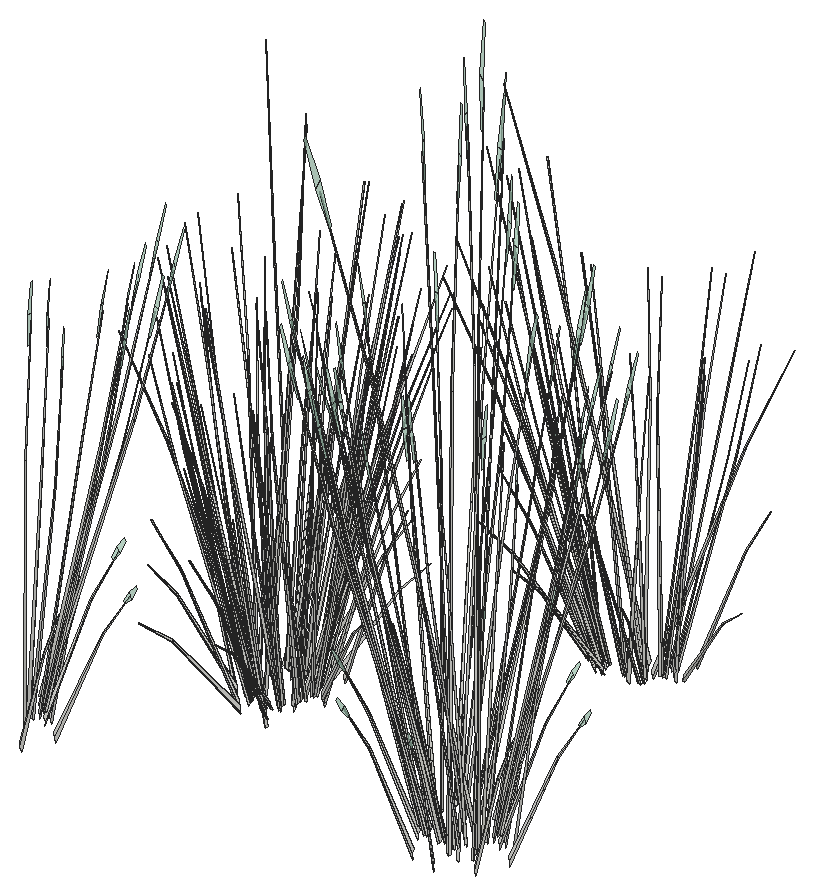
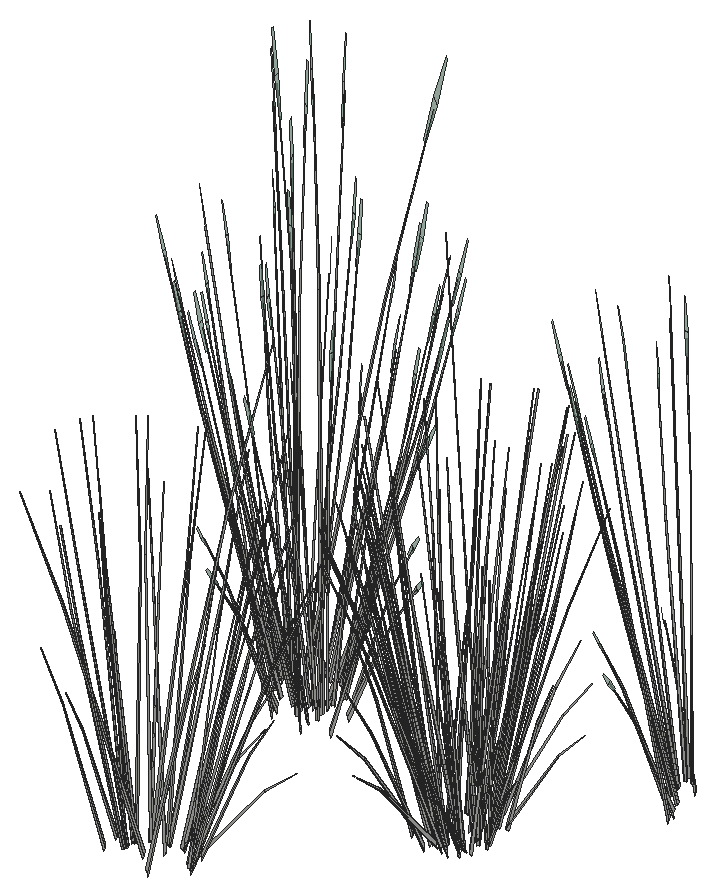
# SketchUp Ruby script. Lengths in inches.
U = 1.inch
M = Sketchup.active_model
def pt(a) = Geom::Point3d.new(a.map { |v| v * U })
def face(e, loops, mat)
  f = e.add_face(loops[0].map { |a| pt(a) })
  loops[1..].each { |l| e.add_face(l.map { |a| pt(a) }).erase! }
  f.material = f.back_material = mat if mat
  f
end
# faces: each face lists its corners as indices into pts; further lists are holes
def faces(e, pts, list, mat = nil) = list.each { |f| face(e, (f[0].is_a?(Array) ? f : [f]).map { |l| l.map { |i| pts[i] } }, mat) }
# xy, xz, yz: faces in a plane at the given z, y or x. An outline is a flat list of corners, or four numbers for a rectangle; further outlines are holes
def ring(l) = l.size == 4 ? [[l[0], l[1]], [l[2], l[1]], [l[2], l[3]], [l[0], l[3]]] : l.each_slice(2).to_a
def flat(e, list, mat, &to3) = list.each { |f| face(e, (f[0].is_a?(Array) ? f : [f]).map { |l| ring(l).map { |u, v| to3.(u, v) } }, mat) }
def xy(e, z, list, mat = nil) = flat(e, list, mat) { |x, y| [x, y, z] }
def xz(e, y, list, mat = nil) = flat(e, list, mat) { |x, z| [x, y, z] }
def yz(e, x, list, mat = nil) = flat(e, list, mat) { |y, z| [x, y, z] }
def lines(e, pts, list) = list.each { |a, b| e.add_line(pt(pts[a]), pt(pts[b])) }
# prism: a flat outline (further loops are holes) pulled along v
def prism(e, loops, v, mat = nil)
  f = face(e, loops, mat); d = Geom::Vector3d.new(v.map { |x| x * U })
  f.pushpull(f.normal.samedirection?(d) ? d.length : -d.length)
end
def box(e, o, s, mat = nil) = prism(e, [[o, [o[0] + s[0], o[1], o[2]], [o[0] + s[0], o[1] + s[1], o[2]], [o[0], o[1] + s[1], o[2]]]], [0, 0, s[2]], mat)
def at(x, y, z, deg = 0) = Geom::Transformation.translation(pt([x, y, z])) * Geom::Transformation.rotation(ORIGIN, Z_AXIS, deg.degrees)
def axes(o, x, y, z) = Geom::Transformation.new([*x, 0, *y, 0, *z, 0, *pt(o).to_a, 1])
def part(name) = M.definitions.add(name)
# library, detail: a bought-in or finely detailed component or shape, given as its bounding box
def library(name, o, s) = part(name).tap { |d| box(d.entities, o, s) }
def detail(e, o, s) = box(e.add_group.entities, o, s)
def put(e, d, t, mat = nil) = e.add_instance(d, t).tap { |i| i.material = mat if mat }
def group(e, t, mat = nil) = e.add_group.tap { |g| g.transformation = t; g.material = mat if mat }.entities
root = M.entities
M.materials.add("LightPink_Translucent").color = [175, 214, 192]
M.materials["LightPink_Translucent"].alpha = 0.75
c1 = part("blade")
p = [[2.15,0.21,22],[0,0.17,0],[0.09,0.45,0],[2.18,0.31,22],[2.29,0.31,22],[0.38,0.45,0],
  [2.48,0.24,33],[2.49,0.24,33],[2.48,0.22,33]]
faces(c1.entities,p,[[0,1,2,3],[4,5,2,3],[6,3,4,7],[8,0,3,6]])
c2 = part("seeds")
p = [[0.3,-0.1,1.38],[-0.01,-0.03,1.59],[-0.01,-0.03,0.03],[0.14,-0.07,-0.07],[0.29,-0.03,3],[0.15,0.01,3.11]]
faces(c2.entities,p,[[0,1,2,3],[1,0,4,5]],"LightPink_Translucent")
c3 = part("blade with seeds")
put(c3.entities,c1,at(0,0,0))
put(c3.entities,c2,axes([2.4,0.25,30.99],[1.5799,-0.05474,1.17369],[-0.12525,1.92788,0.29478],[-0.07173,-0.02425,1.56792]))
c4 = part("blade with seeds\#1")
put(c4.entities,c1,at(0,0,0))
put(root,c3,axes([465.16,230.9,141.8],[0.24965,-0.35138,-0.64651],[0.43748,0.24972,0.07802],[0.14906,-0.12731,0.91455]))
put(root,c3,axes([465.14,230.74,141.52],[-0.12278,-0.40663,-0.465],[0.46497,-0.07113,-0.36018],[0.13325,-0.10922,0.88973]))
put(root,c3,axes([465.71,229.93,139.78],[-0.15919,0.2267,1.04523],[-0.13683,-0.30457,0.76796],[0.13148,-0.07632,0.23022]))
put(root,c3,axes([465.49,230.78,141.38],[0.41603,-0.06364,-0.32227],[0.10985,0.36383,0.41605],[0.11922,-0.09772,0.79608]))
put(root,c3,axes([465.36,231.64,141.52],[0.12948,-0.40508,-0.465],[0.44393,0.13885,-0.36018],[0.17873,-0.03714,0.88973]))
put(root,c3,axes([465.28,231.79,141.8],[0.41997,-0.19668,-0.64651],[0.23405,0.40486,0.07802],[0.20292,-0.04599,0.91455]))
put(root,c3,axes([491.3125,234.65,141.7],[-0.22811,-0.3621,-0.64651],[0.46957,-0.2018,0.07802],[-0.05334,-0.17496,0.91455]))
put(root,c3,axes([492.26,235,141.7],[0.01244,-0.41193,-0.64651],[0.52368,0.02767,0.07802],[0.05527,-0.17451,0.91455]))
put(root,c3,axes([491.36,234.34,141.29],[0.14409,-0.34247,-0.32227],[0.42037,0.09989,0.41605],[-0.03855,-0.13788,0.79608]))
put(root,c3,axes([465.63,231.82,141.38],[0.3972,0.12423,-0.32227],[-0.11585,0.36244,0.41605],[0.15992,-0.03323,0.79608]))
put(root,c3,axes([491.14,234.57,141.43],[-0.46982,-0.11164,-0.465],[0.16104,-0.38276,-0.36018],[-0.04308,-0.1541,0.88973]))
put(root,c3,axes([491.43,233.62,139.6875],[0.06131,0.25968,1.04523],[-0.34012,-0.14383,0.76796],[0.0366,-0.13297,0.23022]))
put(root,c3,axes([492.16,234.86,141.43],[-0.34214,-0.29922,-0.465],[0.36143,-0.26205,-0.36018],[0.05206,-0.15203,0.88973]))
put(root,c3,axes([492.48,234.75,141.29],[0.32338,-0.23447,-0.32227],[0.30612,0.26773,0.41605],[0.04658,-0.13603,0.79608]))
put(root,c3,axes([489.68,233.93,139.6875],[0.24931,0.155,1.04523],[-0.36309,0.09317,0.76796],[-0.07769,-0.11912,0.23022]))
put(root,c3,axes([490.29,234.75,141.7],[-0.40754,-0.21525,-0.64651],[0.28963,-0.37719,0.07802],[-0.14765,-0.12852,0.91455]))
put(root,c3,axes([490.14,234.47,141.29],[-0.07382,-0.3587,-0.32227],[0.42197,-0.09472,0.41605],[-0.11334,-0.10279,0.79608]))
put(root,c3,axes([466.47,231.9,139.78],[-0.2953,0.07352,1.04523],[0.139,-0.30384,0.76796],[0.15666,0.02079,0.23022]))
put(root,c3,axes([490.1,234.76,141.43],[-0.47162,0.10586,-0.465],[-0.0825,-0.4009,-0.36018],[-0.12667,-0.11489,0.88973]))
put(root,c3,axes([492.88,235.72,141.7],[0.24965,-0.35138,-0.64651],[0.43748,0.24972,0.07802],[0.14906,-0.12731,0.91455]))
put(root,c3,axes([492.87,235.55,141.43],[-0.12278,-0.40663,-0.465],[0.46497,-0.07113,-0.36018],[0.13325,-0.10922,0.88973]))
put(root,c3,axes([491.26,237.19,140.2],[0.41302,0.17958,1.37647],[-0.40462,0.38687,0.54432],[-0.18124,-0.22929,1.15394]))
put(root,c3,axes([464.86,232.6,141.8],[0.47777,0.01072,-0.64651],[-0.03209,0.45152,0.07802],[0.2024,0.04765,0.91455]))
put(root,c3,axes([493.4375,234.74,139.6875],[-0.15919,0.2267,1.04523],[-0.13683,-0.30457,0.76796],[0.13148,-0.07632,0.23022]))
put(root,c3,axes([493.21,235.6,141.29],[0.41603,-0.06364,-0.32227],[0.10985,0.36383,0.41605],[0.11922,-0.09772,0.79608]))
put(root,c3,axes([489.17,235.1,141.29],[-0.27194,-0.27882,-0.32227],[0.31051,-0.26394,0.41605],[-0.15777,-0.04016,0.79608]))
put(root,c3,axes([465.15,232.79,141.38],[0.27194,0.27882,-0.32227],[-0.31051,0.26394,0.41605],[0.15777,0.04016,0.79608]))
put(root,c3,axes([489.45,235.28,141.7],[-0.47777,-0.01072,-0.64651],[0.03209,-0.45152,0.07802],[-0.2024,-0.04765,0.91455]))
put(root,c3,axes([464.83,232.95,139.78],[-0.2691,-0.12805,1.04523],[0.34747,-0.13011,0.76796],[0.09372,0.11021,0.23022]))
put(root,c3,axes([489.3,235.375,141.43],[-0.34704,0.29499,-0.465],[-0.30393,-0.31162,-0.36018],[-0.17633,-0.04488,0.88973]))
put(root,c3,axes([488.51,235.76,139.6875],[0.30513,-0.03187,1.04523],[-0.19355,0.28077,0.76796],[-0.15079,-0.04212,0.23022]))
put(root,c3,axes([490.67,236.02,139.64],[-0.519,0.02749,0.40713],[-0.04694,-0.45634,-0.19594],[0.09291,-0.04625,1.30716]))
put(root,c3,axes([464.22,233.125,141.52],[0.47162,-0.10586,-0.465],[0.0825,0.4009,-0.36018],[0.12667,0.11489,0.88973]))
put(root,c3,axes([493.08,236.46,141.43],[0.12948,-0.40508,-0.465],[0.44393,0.13885,-0.36018],[0.17873,-0.03714,0.88973]))
put(root,c3,axes([464.875,233.53,139.69],[-0.30649,-0.01397,0.95605],[0.2024,-0.29664,0.52785],[0.12108,0.10539,0.74993]))
put(root,c3,axes([490.55,236.58,139.64],[-0.23189,0.40128,0.40713],[-0.48183,-0.19312,-0.19594],[0,-0.0925,1.30716]))
put(root,c3,axes([493,236.6,141.7],[0.41997,-0.19668,-0.64651],[0.23405,0.40486,0.07802],[0.20292,-0.04599,0.91455]))
put(root,c3,axes([491.29,235.84,139.64],[-0.28711,-0.37379,0.40713],[0.43489,-0.26322,-0.19594],[0.09291,0.04625,1.30716]))
put(root,c3,axes([493.36,236.64,141.29],[0.3972,0.12423,-0.32227],[-0.11585,0.36244,0.41605],[0.15992,-0.03323,0.79608]))
put(root,c3,axes([488.6875,236.0625,141.29],[-0.3972,-0.12423,-0.32227],[0.11585,-0.36244,0.41605],[-0.15992,0.03323,0.79608]))
put(root,c4,axes([473.13,239.73,140.59],[-0.05804,-0.06898,1.43516],[-0.35603,0.0883,-0.22697],[-0.0675,-0.17309,0.1151]))
put(root,c3,axes([489.9,236,140.21],[0.13585,-0.06442,1.61128],[0.04685,0.4498,0.1261],[-0.29426,0.05969,0.57588]))
put(root,c3,axes([494.2,236.71,139.6875],[-0.2953,0.07352,1.04523],[0.139,-0.30384,0.76796],[0.15666,0.02079,0.23022]))
put(root,c4,axes([474.7,240.09,140.58],[-0.03336,0.04495,1.45516],[-0.35758,-0.09833,-0.1375],[-0.02285,-0.17707,0.25751]))
put(root,c4,axes([473.15,241.95,139.9],[0.00863,0.2062,1.40588],[-0.37404,-0.13679,0.11368],[0.02314,-0.29386,0.601]))
put(root,c3,axes([491.79,236.21,139.64],[0.23189,-0.40128,0.40713],[0.48183,0.19312,-0.19594],[0,0.0925,1.30716]))
put(root,c3,axes([488.96,236.25,141.43],[-0.12948,0.40508,-0.465],[-0.44393,-0.13885,-0.36018],[-0.17873,0.03714,0.88973]))
put(root,c3,axes([493.6875,237.65,140.75],[-0.09148,-0.37435,-0.03177],[0.43236,-0.08606,-0.14407],[0.09029,0.02373,0.47519]))
put(root,c4,axes([473.53,240.82,140.43],[0.1063,-0.41315,-0.29052],[0.31012,0.1205,0.37506],[-0.02844,-0.16634,0.71765]))
put(root,c3,axes([491.67,236.76,139.64],[0.519,-0.02749,0.40713],[0.04694,0.45634,-0.19594],[-0.09291,0.04625,1.30716]))
put(root,c4,axes([474.16,241.21,140.59],[-0.00644,-0.10664,1.43516],[-0.29603,-0.29251,-0.22697],[0.03908,-0.18969,0.1151]))
put(root,c4,axes([473.67,241.08,140.85],[-0.34504,0.25013,-0.09976],[-0.16956,-0.44394,-0.55369],[-0.04552,-0.18708,0.84132]))
put(root,c4,axes([473.57,240.92,140.6],[0.34743,0.14045,0.39379],[-0.1188,0.46175,0.3247],[-0.02088,-0.18159,0.81485]))
put(root,c4,axes([474.39,241.65,140.85],[-0.38751,-0.02662,-0.09976],[0.01059,-0.50399,-0.55369],[0.02692,-0.19411,0.84132]))
put(root,c4,axes([473.66,240.88,140.6],[0.25981,-0.18259,0.05275],[0.12717,0.33295,0.41527],[-0.02509,-0.14677,0.63322]))
put(root,c4,axes([472.76,239.97,140.58],[-0.00289,0.06493,1.45516],[-0.31009,0.26964,-0.1375],[-0.10196,-0.10828,0.25751]))
put(root,c4,axes([472.64,240.97,140.43],[-0.05446,-0.43273,-0.29052],[0.31131,-0.11427,0.37506],[-0.08362,-0.12401,0.71765]))
put(root,c4,axes([474.36,241.32,140.43],[0.23857,-0.28286,-0.29052],[0.22584,0.32298,0.37506],[0.03436,-0.1641,0.71765]))
put(root,c3,axes([492.59,237.42,141.7],[0.47777,0.01072,-0.64651],[-0.03209,0.45152,0.07802],[0.2024,0.04765,0.91455]))
put(root,c4,axes([473.75,242.34,139.9],[-0.06565,0.18466,1.40588],[-0.27542,-0.38215,0.11368],[0.12424,-0.23818,0.601]))
put(root,c4,axes([472.71,241.03,140.6],[0.35069,-0.12329,0.39379],[0.06086,0.48364,0.3247],[-0.08248,-0.14254,0.81485]))
put(root,c4,axes([472.77,240.93,140.6],[0.16025,-0.34128,0.05275],[0.22821,0.1987,0.41527],[-0.07378,-0.10942,0.63322]))
put(root,c3,axes([488.08,237.98,139.6875],[0.19918,-0.20183,1.04523],[0.0786,0.31952,0.76796],[-0.14394,0.05721,0.23022]))
put(root,c3,axes([492.875,237.61,141.29],[0.27194,0.27882,-0.32227],[-0.31051,0.26394,0.41605],[0.15777,0.04016,0.79608]))
put(root,c3,axes([488.83,237.11,141.29],[-0.41603,0.06364,-0.32227],[-0.10985,-0.36383,0.41605],[-0.11922,0.09772,0.79608]))
put(root,c4,axes([474.4,240.48,139.94],[-0.32031,0.09515,-0.02864],[-0.07364,-0.44972,-0.12987],[0.02031,-0.09391,0.42837]))
put(root,c4,axes([474.36,241.43,140.6],[0.25108,0.36656,0.39379],[-0.26664,0.31614,0.3247],[0.04631,-0.17198,0.81485]))
put(root,c4,axes([474.45,241.47,140.6],[0.28975,0.02503,0.05275],[-0.00794,0.378,0.41527],[0.03032,-0.1448,0.63322]))
put(root,c4,axes([472.85,241.1,140.85],[-0.21011,0.45986,-0.09976],[-0.30427,-0.26493,-0.55369],[-0.10577,-0.12992,0.84132]))
put(root,c3,axes([492.56,237.77,139.6875],[-0.2691,-0.12805,1.04523],[0.34747,-0.13011,0.76796],[0.09372,0.11021,0.23022]))
put(root,c4,axes([474.81,242.64,140.85],[-0.32616,-0.29624,-0.09976],[0.1879,-0.42901,-0.55369],[0.09215,-0.14913,0.84132]))
put(root,c3,axes([489.18,237.15,141.43],[0.12278,0.40663,-0.465],[-0.46497,0.07113,-0.36018],[-0.13325,0.10922,0.88973]))
put(root,c3,axes([491.9,236.33,139.76],[-0.01306,-0.4193,1.28558],[0.59089,0.10869,0.54432],[-0.13975,0.22943,1.21348]))
put(root,c4,axes([471.95,242.57,139.9],[0.13097,0.09256,1.40588],[-0.27104,0.38832,0.11368],[-0.16893,-0.17518,0.601]))
put(root,c3,axes([491.95,237.94,141.43],[0.47162,-0.10586,-0.465],[0.0825,0.4009,-0.36018],[0.12667,0.11489,0.88973]))
put(root,c3,axes([492.6,238.35,139.6],[-0.30649,-0.01397,0.95605],[0.2024,-0.29664,0.52785],[0.12108,0.10539,0.74993]))
put(root,c4,axes([471.58,241.2,140.59],[-0.07584,0.0048,1.43516],[-0.21918,0.40531,-0.22697],[-0.13286,-0.06266,0.1151]))
put(root,c4,axes([472,241.74,140.6],[0.25999,-0.354,0.39379],[0.22422,0.37594,0.3247],[-0.12198,-0.0653,0.81485]))
put(root,c4,axes([472.02,241.61,140.6],[0.01775,-0.40853,0.05275],[0.2681,0.0112,0.41527],[-0.1027,-0.04275,0.63322]))
put(root,c4,axes([472.89,242.3,140.39],[-0.19798,0.42958,1.1344],[-0.30825,-0.45359,0.48946],[0.18577,-0.1386,1.09651]))
put(root,c4,axes([471.92,241.73,140.43],[-0.20062,-0.33637,-0.29052],[0.22908,-0.31842,0.37506],[-0.11639,-0.04845,0.71765]))
put(root,c4,axes([475.08,243.02,140.58],[-0.04613,-0.00147,1.45516],[-0.20353,-0.42603,-0.1375],[0.07265,-0.14798,0.25751]))
put(root,c3,axes([489.56,237.95,141.29],[-0.32338,0.23447,-0.32227],[-0.30612,-0.26773,0.41605],[-0.04658,0.13603,0.79608]))
put(root,c3,axes([489.77,238.86,139.6875],[-0.01237,-0.2648,1.04523],[0.30908,0.18886,0.76796],[-0.06079,0.12621,0.23022]))
put(root,c3,axes([489.89,237.84,141.72],[0.34214,0.29922,-0.51615],[-0.36143,0.26205,-0.3998],[-0.05206,0.15203,0.9876]))
put(root,c4,axes([474.13,243.1,139.9],[-0.12234,0.11364,1.40588],[-0.103,-0.52511,0.11368],[0.19206,-0.11868,0.601]))
put(root,c4,axes([474.86,242.43,140.6],[0.08745,0.49445,0.39379],[-0.34303,0.08581,0.3247],[0.1011,-0.11629,0.81485]))
put(root,c3,axes([490.9,238.13,141.43],[0.46982,0.11164,-0.465],[-0.16104,0.38276,-0.36018],[0.04308,0.1541,0.88973]))
put(root,c4,axes([474.93,242.53,140.6],[0.24206,0.22594,0.05275],[-0.14093,0.32175,0.41527],[0.07761,-0.10402,0.63322]))
put(root,c3,axes([490.6875,238.37,141.29],[-0.14409,0.34247,-0.32227],[-0.42037,-0.09989,0.41605],[0.03855,0.13788,0.79608]))
put(root,c3,axes([489.78,237.7,142.03],[-0.01244,0.41193,-0.71763],[-0.52368,-0.02767,0.0866],[-0.05527,0.17451,1.01516]))
put(root,c4,axes([472.15,241.7,140.85],[-0.01888,0.54637,-0.09976],[-0.35746,-0.01493,-0.55369],[-0.13767,-0.03795,0.84132]))
put(root,c3,axes([490.73,238.06,141.7],[0.22811,0.3621,-0.64651],[-0.46957,0.2018,0.07802],[0.05334,0.17496,0.91455]))
put(root,c4,axes([471.31,241.31,140.58],[0.0291,0.05049,1.45516],[-0.09819,0.49465,-0.1375],[-0.12701,0.01791,0.25751]))
put(root,c4,axes([474.82,243.79,140.85],[-0.17741,-0.48648,-0.09976],[0.31487,-0.23906,-0.55369],[0.13269,-0.06419,0.84132]))
put(root,c3,axes([489.6,238.28,140.23],[0.0105,-0.22989,1.40454],[0.4723,0.12143,0.19409],[-0.04092,0.24501,0.66323]))
put(root,c4,axes([471.63,242.85,140.6],[0.09962,-0.48986,0.39379],[0.3275,0.16751,0.3247],[-0.12879,0.02944,0.81485]))
put(root,c4,axes([471.61,242.72,140.6],[-0.1295,-0.36632,0.05275],[0.23615,-0.1793,0.41527],[-0.1041,0.03538,0.63322]))
put(root,c4,axes([475.53,243.91,140.59],[0.06136,-0.06302,1.43516],[0.02411,-0.50855,-0.22697],[0.13532,-0.05114,0.1151]))
put(root,c4,axes([471.5625,242.9,140.43],[-0.29303,-0.14987,-0.29052],[0.08547,-0.43725,0.37506],[-0.11798,0.04009,0.71765]))
put(root,c4,axes([475.01,243.6,140.43],[0.29303,0.14987,-0.29052],[-0.08547,0.43725,0.37506],[0.11798,-0.04009,0.71765]))
put(root,c4,axes([474.97,243.78,140.6],[0.1295,0.36632,0.05275],[-0.23615,0.1793,0.41527],[0.1041,-0.03538,0.63322]))
put(root,c4,axes([474.19,244.03,139.9],[-0.14625,0.01217,1.40588],[0.09702,-0.52737,0.11368],[0.20842,0.03262,0.601]))
put(root,c4,axes([471.75,242.71,140.85],[0.17741,0.48648,-0.09976],[-0.31487,0.23906,-0.55369],[-0.13269,0.06419,0.84132]))
put(root,c4,axes([474.42,244.8,141.15],[0.01888,-0.54637,-0.11073],[0.35746,0.01493,-0.6146],[0.13767,0.03795,0.93387]))
put(root,c4,axes([474.56,244.43,140.82],[0.25603,-0.35588,-0.4653],[0.22422,0.37594,-0.36041],[0.13008,0.05415,0.89031]))
put(root,c4,axes([470.92,243.48,140.59],[-0.05342,0.07604,1.43516],[0.03387,0.50744,-0.22697],[-0.12778,0.08099,0.1151]))
put(root,c4,axes([474.9375,244.72,139.48],[-0.19671,-0.01092,1.26617],[0.1039,-0.49126,0.17497],[0.20964,0.04257,0.59789]))
put(root,c4,axes([471.64,243.97,140.6],[-0.24206,-0.22594,0.05275],[0.14093,-0.32175,0.41527],[-0.07761,0.10402,0.63322]))
put(root,c4,axes([474,243,139.45],[0.15365,-0.4296,1.24087],[0.33102,0.42086,0.4907],[-0.19619,0.18851,1.04025]))
put(root,c4,axes([475.37,245.97,140.58],[-0.02301,-0.0564,1.45516],[0.15302,-0.46615,-0.1375],[0.12741,0.01095,0.25751]))
put(root,c4,axes([471.67,244.16,140.43],[-0.30692,0.07678,-0.29052],[-0.08104,-0.43892,0.37506],[-0.08795,0.11789,0.71765]))
put(root,c4,axes([474.65,244.77,140.43],[0.20062,0.33637,-0.29052],[-0.22908,0.31842,0.37506],[0.11639,0.04845,0.71765]))
put(root,c4,axes([474.55,244.89,140.6],[-0.01775,0.40853,0.05275],[-0.2681,-0.0112,0.41527],[0.1027,0.04275,0.63322]))
put(root,c4,axes([474.58,244.76,140.6],[-0.25999,0.354,0.39379],[-0.22422,-0.37594,0.3247],[0.12198,0.0653,0.81485]))
put(root,c4,axes([471.74,244.35,139.9],[0.12234,-0.11364,1.40588],[0.103,0.52511,0.11368],[-0.19206,0.11868,0.601]))
put(root,c4,axes([470.75,244,140.58],[0.04567,0.00927,1.45516],[0.16576,0.45742,-0.1375],[-0.08473,0.1346,0.25751]))
put(root,c4,axes([473.72,245.4,140.85],[0.21011,-0.45986,-0.09976],[0.30427,0.26493,-0.55369],[0.10577,0.12992,0.84132]))
put(root,c4,axes([471.62,243.87,141.17],[0.3653,0.33178,-0.11173],[-0.21045,0.48049,-0.62013],[-0.10321,0.16702,0.94228]))
put(root,c4,axes([472.12,245.03,140.6],[-0.28975,-0.02503,0.05275],[0.00794,-0.378,0.41527],[-0.03032,0.1448,0.63322]))
put(root,c4,axes([474.59,245.93,140.59],[0.0754,0.01236,1.43516],[0.26232,-0.35069,-0.22697],[0.12405,0.09181,0.1151]))
put(root,c4,axes([473.92,244.87,139.9],[-0.13097,-0.09256,1.40588],[0.27104,-0.38832,0.11368],[0.16893,0.17518,0.601]))
put(root,c4,axes([473.8,245.57,140.6],[-0.16025,0.34128,0.05275],[-0.22821,-0.1987,0.41527],[0.07378,0.10942,0.63322]))
put(root,c4,axes([473.87,245.47,140.6],[-0.35069,0.12329,0.39379],[-0.06086,-0.48364,0.3247],[0.08248,0.14254,0.81485]))
put(root,c4,axes([473.63,244.78,139.9],[-0.11708,-0.12417,1.40588],[0.31602,-0.31352,0.11368],[0.14392,0.21504,0.601]))
put(root,c4,axes([472.21,245.18,140.43],[-0.23857,0.28286,-0.29052],[-0.22584,-0.32298,0.37506],[-0.03436,0.1641,0.71765]))
put(root,c4,axes([473.93,245.53,140.43],[0.05446,0.43273,-0.29052],[-0.31131,0.11427,0.37506],[0.08362,0.12401,0.71765]))
put(root,c4,axes([472.91,245.62,140.6],[-0.25981,0.18259,0.05275],[-0.12717,-0.33295,0.41527],[0.02509,0.14677,0.63322]))
put(root,c4,axes([472.18,244.86,140.85],[0.38751,0.02662,-0.09976],[-0.01059,0.50399,-0.55369],[-0.02692,0.19411,0.84132]))
put(root,c4,axes([473,245.58,140.6],[-0.34743,-0.14045,0.39379],[0.1188,-0.46175,0.3247],[0.02088,0.18159,0.81485]))
put(root,c4,axes([472.9,245.42,140.85],[0.34504,-0.25013,-0.09976],[0.16956,0.44394,-0.55369],[0.04552,0.18708,0.84132]))
put(root,c4,axes([471.51,245.14,140.59],[-0.00269,0.10696,1.43516],[0.26896,0.34054,-0.22697],[-0.05496,0.1817,0.1151]))
put(root,c4,axes([471.74,245.55,140.58],[0.03803,-0.03685,1.45516],[0.34183,0.17767,-0.1375],[0.00247,0.17994,0.25751]))
put(root,c4,axes([473.61,246.84,140.58],[0.01022,-0.06344,1.45516],[0.33667,-0.19627,-0.1375],[0.08837,0.12987,0.25751]))
put(root,c4,axes([473.04,245.68,140.43],[-0.1063,0.41315,-0.29052],[-0.31012,-0.1205,0.37506],[0.02844,0.16634,0.71765]))
put(root,c4,axes([472.12,245.11,139.9],[0.06565,-0.18466,1.40588],[0.27542,0.38215,0.11368],[-0.12424,0.23818,0.601]))
put(root,c4,axes([473.25,245.9375,140.59],[0.04947,0.08118,1.43516],[0.36146,-0.00691,-0.22697],[0.04701,0.18608,0.1151]))
put(root,c4,axes([473.375,245.41,139.9],[-0.0806,-0.17249,1.40588],[0.37244,-0.14522,0.11368],[0.08417,0.2708,0.601]))
put(root,c4,axes([472.72,245.5,139.9],[-0.00863,-0.2062,1.40588],[0.37404,0.13679,0.11368],[-0.02314,0.29386,0.601]))
put(root,c4,axes([485.03,256.21,139.9],[0.11364,0.12234,1.40588],[-0.52511,0.103,0.11368],[-0.11868,-0.19206,0.601]))
put(root,c4,axes([485.9,255.4,140.59],[-0.07604,-0.05342,1.43516],[-0.50744,0.03387,-0.22697],[-0.08099,-0.12778,0.1151]))
put(root,c4,axes([488.07,255.79,140.58],[-0.05049,0.0291,1.45516],[-0.49465,-0.09819,-0.1375],[-0.01791,-0.12701,0.25751]))
put(root,c4,axes([488.18,256.06,140.59],[-0.0048,-0.07584,1.43516],[-0.40531,-0.21918,-0.22697],[0.06266,-0.13286,0.1151]))
put(root,c4,axes([486.8,256.43,139.9],[-0.09256,0.13097,1.40588],[-0.38832,-0.27104,0.11368],[0.17518,-0.16893,0.601]))
put(root,c4,axes([486.47,256.04,140.43],[0.14987,-0.29303,-0.29052],[0.43725,0.08547,0.37506],[-0.04009,-0.11798,0.71765]))
put(root,c4,axes([485.375,255.23,140.58],[-0.00927,0.04567,1.45516],[-0.45742,0.16576,-0.1375],[-0.1346,-0.08473,0.25751]))
put(root,c4,axes([486.67,256.23,140.85],[-0.48648,0.17741,-0.09976],[-0.23906,-0.31487,-0.55369],[-0.06419,-0.13269,0.84132]))
put(root,c4,axes([486.53,256.11,140.6],[0.48986,0.09962,0.39379],[-0.16751,0.3275,0.3247],[-0.02944,-0.12879,0.81485]))
put(root,c4,axes([487.68,256.625,140.85],[-0.54637,-0.01888,-0.09976],[0.01493,-0.35746,-0.55369],[0.03795,-0.13767,0.84132]))
put(root,c4,axes([485.21,256.15,140.43],[-0.07678,-0.30692,-0.29052],[0.43892,-0.08104,0.37506],[-0.11789,-0.08795,0.71765]))
put(root,c4,axes([487.64,256.4,140.43],[0.33637,-0.20062,-0.29052],[0.31842,0.22908,0.37506],[0.04845,-0.11639,0.71765]))
put(root,c4,axes([485.4,256.12,140.6],[0.22594,-0.24206,0.05275],[0.32175,0.14093,0.41527],[-0.10402,-0.07761,0.63322]))
put(root,c4,axes([484.27,256.6,139.9],[0.18466,0.06565,1.40588],[-0.38215,0.27542,0.11368],[-0.23818,-0.12424,0.601]))
put(root,c4,axes([485.5,256.1,141.17],[-0.33178,0.3653,-0.11173],[-0.48049,-0.21045,-0.62013],[-0.16702,-0.10321,0.94228]))
put(root,c4,axes([487.64,256.48,140.6],[0.354,0.25999,0.39379],[-0.37594,0.22422,0.3247],[0.0653,-0.12198,0.81485]))
put(root,c4,axes([484.23,255.99,140.59],[-0.10696,-0.00269,1.43516],[-0.34054,0.26896,-0.22697],[-0.1817,-0.05496,0.1151]))
put(root,c4,axes([488.27,257.33,140.85],[-0.45986,-0.21011,-0.09976],[0.26493,-0.30427,-0.55369],[0.12992,-0.10577,0.84132]))
put(root,c4,axes([489.41,257.24,140.58],[-0.06493,-0.00289,1.45516],[-0.26964,-0.31009,-0.1375],[0.10828,-0.10196,0.25751]))
put(root,c4,axes([486.375,258.48,139.45],[0.4296,0.15365,1.24087],[-0.42086,0.33102,0.4907],[-0.18851,-0.19619,1.04025]))
put(root,c4,axes([484.2,256.69,140.43],[-0.28286,-0.23857,-0.29052],[0.32298,-0.22584,0.37506],[-0.1641,-0.03436,0.71765]))
put(root,c4,axes([488.4,257.12,140.43],[0.43273,-0.05446,-0.29052],[0.11427,0.31131,0.37506],[0.12401,-0.08362,0.71765]))
put(root,c4,axes([488.35,257.19,140.6],[0.12329,0.35069,0.39379],[-0.48364,0.06086,0.3247],[0.14254,-0.08248,0.81485]))
put(root,c4,axes([488.44,257.25,140.6],[0.34128,0.16025,0.05275],[-0.1987,0.22821,0.41527],[0.10942,-0.07378,0.63322]))
put(root,c4,axes([489.65,257.61,140.59],[0.06898,-0.05804,1.43516],[-0.0883,-0.35603,-0.22697],[0.17309,-0.0675,0.1151]))
put(root,c4,axes([483.82,256.22,140.58],[0.03685,0.03803,1.45516],[-0.17767,0.34183,-0.1375],[-0.17994,0.00247,0.25751]))
put(root,c4,axes([484.52,256.66,140.85],[-0.02662,0.38751,-0.09976],[-0.50399,-0.01059,-0.55369],[-0.19411,-0.02692,0.84132]))
put(root,c4,axes([488.29,258.15,140.85],[-0.25013,-0.34504,-0.09976],[0.44394,-0.16956,-0.55369],[0.18708,-0.04552,0.84132]))
put(root,c4,axes([483.88,257.2,139.9],[0.2062,-0.00863,1.40588],[-0.13679,0.37404,0.11368],[-0.29386,-0.02314,0.601]))
put(root,c4,axes([483.79,257.48,140.6],[0.14045,-0.34743,0.39379],[0.46175,0.1188,0.3247],[-0.18159,0.02088,0.81485]))
put(root,c4,axes([483.7,257.52,140.43],[-0.41315,-0.1063,-0.29052],[0.1205,-0.31012,0.37506],[-0.16634,0.02844,0.71765]))
put(root,c4,axes([488.55,258.01,140.43],[0.41315,0.1063,-0.29052],[-0.1205,0.31012,0.37506],[0.16634,-0.02844,0.71765]))
put(root,c4,axes([487.43,257.63,139.9],[-0.2062,0.00863,1.40588],[0.13679,-0.37404,0.11368],[0.29386,0.02314,0.601]))
put(root,c4,axes([488.49,258.14,140.6],[0.18259,0.25981,0.05275],[-0.33295,0.12717,0.41527],[0.14677,-0.02509,0.63322]))
put(root,c4,axes([488.46,258.05,140.6],[-0.14045,0.34743,0.39379],[-0.46175,-0.1188,0.3247],[0.18159,-0.02088,0.81485]))
put(root,c4,axes([483.96,257.38,140.85],[0.25013,0.34504,-0.09976],[-0.44394,0.16956,-0.55369],[-0.18708,0.04552,0.84132]))
put(root,c4,axes([489.29,259.18,140.58],[-0.04495,-0.03336,1.45516],[0.09833,-0.35758,-0.1375],[0.17707,-0.02285,0.25751]))
